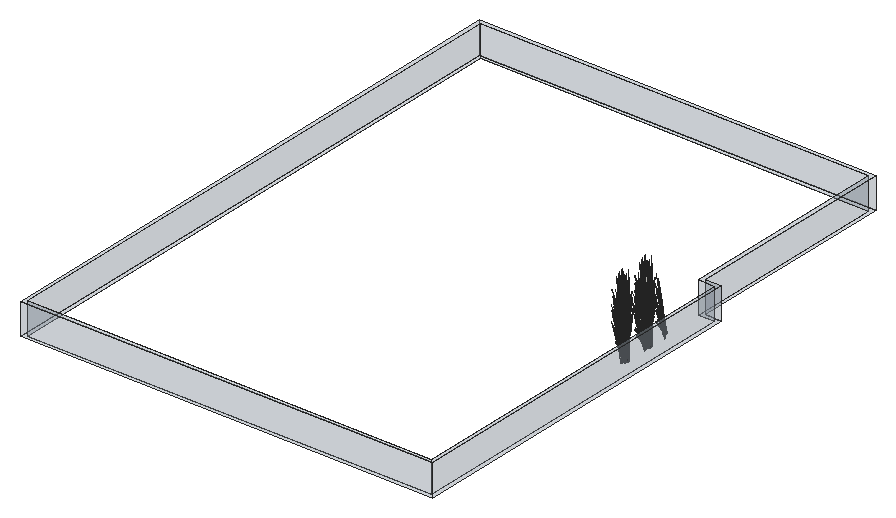
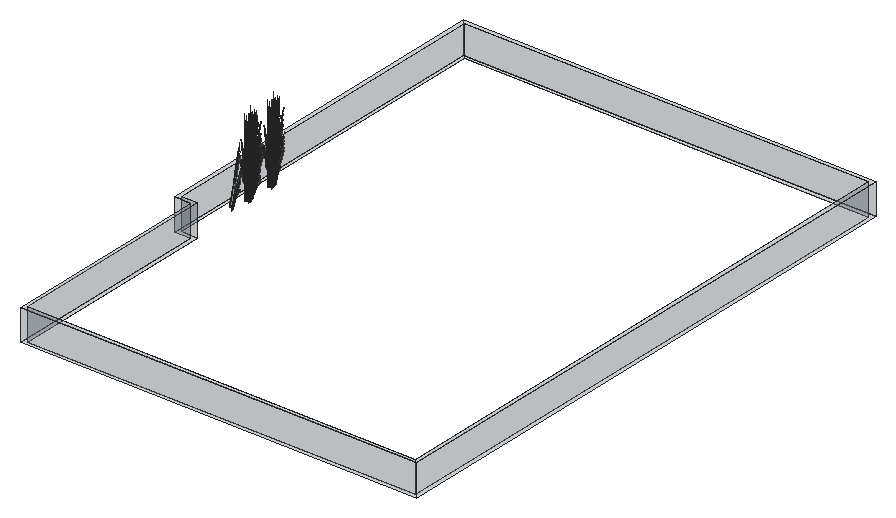
# SketchUp Ruby script. Lengths in inches.
U = 1.inch
M = Sketchup.active_model
def pt(a) = Geom::Point3d.new(a.map { |v| v * U })
def face(e, loops, mat)
  f = e.add_face(loops[0].map { |a| pt(a) })
  loops[1..].each { |l| e.add_face(l.map { |a| pt(a) }).erase! }
  f.material = f.back_material = mat if mat
  f
end
# faces: each face lists its corners as indices into pts; further lists are holes
def faces(e, pts, list, mat = nil) = list.each { |f| face(e, (f[0].is_a?(Array) ? f : [f]).map { |l| l.map { |i| pts[i] } }, mat) }
# xy, xz, yz: faces in a plane at the given z, y or x. An outline is a flat list of corners, or four numbers for a rectangle; further outlines are holes
def ring(l) = l.size == 4 ? [[l[0], l[1]], [l[2], l[1]], [l[2], l[3]], [l[0], l[3]]] : l.each_slice(2).to_a
def flat(e, list, mat, &to3) = list.each { |f| face(e, (f[0].is_a?(Array) ? f : [f]).map { |l| ring(l).map { |u, v| to3.(u, v) } }, mat) }
def xy(e, z, list, mat = nil) = flat(e, list, mat) { |x, y| [x, y, z] }
def xz(e, y, list, mat = nil) = flat(e, list, mat) { |x, z| [x, y, z] }
def yz(e, x, list, mat = nil) = flat(e, list, mat) { |y, z| [x, y, z] }
def lines(e, pts, list) = list.each { |a, b| e.add_line(pt(pts[a]), pt(pts[b])) }
# prism: a flat outline (further loops are holes) pulled along v
def prism(e, loops, v, mat = nil)
  f = face(e, loops, mat); d = Geom::Vector3d.new(v.map { |x| x * U })
  f.pushpull(f.normal.samedirection?(d) ? d.length : -d.length)
end
def box(e, o, s, mat = nil) = prism(e, [[o, [o[0] + s[0], o[1], o[2]], [o[0] + s[0], o[1] + s[1], o[2]], [o[0], o[1] + s[1], o[2]]]], [0, 0, s[2]], mat)
def at(x, y, z, deg = 0) = Geom::Transformation.translation(pt([x, y, z])) * Geom::Transformation.rotation(ORIGIN, Z_AXIS, deg.degrees)
def axes(o, x, y, z) = Geom::Transformation.new([*x, 0, *y, 0, *z, 0, *pt(o).to_a, 1])
def part(name) = M.definitions.add(name)
# library, detail: a bought-in or finely detailed component or shape, given as its bounding box
def library(name, o, s) = part(name).tap { |d| box(d.entities, o, s) }
def detail(e, o, s) = box(e.add_group.entities, o, s)
def put(e, d, t, mat = nil) = e.add_instance(d, t).tap { |i| i.material = mat if mat }
def group(e, t, mat = nil) = e.add_group.tap { |g| g.transformation = t; g.material = mat if mat }.entities
root = M.entities
M.materials.add("Glass_Basic_2").color = [161, 173, 186]
M.materials["Glass_Basic_2"].alpha = 0.25
M.materials.add("LightPink_Translucent").color = [144, 107, 117]
M.materials["LightPink_Translucent"].alpha = 0.75
c1 = part("blade")
p = [[2.15,0.21,22],[0,0.17,0],[0.09,0.45,0],[2.18,0.31,22],[2.29,0.31,22],[0.38,0.45,0],
  [2.48,0.24,33],[2.49,0.24,33],[2.48,0.22,33]]
faces(c1.entities,p,[[0,1,2,3],[4,5,2,3],[6,3,4,7],[8,0,3,6]])
c2 = part("seeds")
p = [[0.3,-0.1,1.38],[-0.01,-0.03,1.59],[-0.01,-0.03,0.03],[0.14,-0.07,-0.07],[0.29,-0.03,3],[0.15,0.01,3.11]]
faces(c2.entities,p,[[0,1,2,3],[1,0,4,5]],"LightPink_Translucent")
c3 = part("blade with seeds")
put(c3.entities,c1,at(0,0,0))
put(c3.entities,c2,axes([2.4,0.25,30.99],[1.5799,-0.05474,1.17369],[-0.12525,1.92788,0.29478],[-0.07173,-0.02425,1.56792]))
g1 = group(root,at(30.57,364.54,1398),"Glass_Basic_2")
prism(g1,[[[0,0,0],[0,434.16,0],[300,434.16,0],[300,273.36,0],[312,273.36,0],[312,0,0]],[[297,431.16,0],[3,431.16,0],[3,3,0],[309,3,0],[309,270.36,0],[297,270.36,0]]],[0,0,24])
put(root,c3,axes([329.46,560.04,1401.875],[0.14639,-0.01056,1.71376],[-0.09712,0.45778,0.13857],[-0.20862,-0.02831,0.73262]))
put(root,c3,axes([329.46,581.76,1401.875],[0.14639,-0.01056,1.71376],[-0.09712,0.45778,0.13857],[-0.20862,-0.02831,0.73262]))
put(root,c3,axes([329.52,560.85,1401.875],[0.12246,-0.09864,1.71376],[0.1031,0.45582,0.13857],[-0.19225,0.10302,0.73262]))
put(root,c3,axes([329.52,582.5625,1401.875],[0.12246,-0.09864,1.71376],[0.1031,0.45582,0.13857],[-0.19225,0.10302,0.73262]))
put(root,c3,axes([329.14,561.625,1400.59],[0.12266,0.03828,1.43002],[0.07906,0.39104,-0.30754],[-0.16661,0.0732,0.61141]))
put(root,c3,axes([329.14,583.34,1400.59],[0.12266,0.03828,1.43002],[0.07906,0.39104,-0.30754],[-0.16661,0.0732,0.61141]))
put(root,c3,axes([330.22,560.37,1401.34],[0.10032,-0.06746,1.77064],[0.0346,0.47103,0.13857],[-0.2173,0.0625,0.63284]))
put(root,c3,axes([330.22,582.09,1401.34],[0.10032,-0.06746,1.77064],[0.0346,0.47103,0.13857],[-0.2173,0.0625,0.63284]))
put(root,c3,axes([329.14,560.6875,1402.72],[-0.05763,0.06055,1.74944],[0.0049,0.44239,-0.27667],[-0.13211,0.05753,0.14031]))
put(root,c3,axes([329.14,582.4,1402.72],[-0.05763,0.06055,1.74944],[0.0049,0.44239,-0.27667],[-0.13211,0.05753,0.14031]))
put(root,c3,axes([329.89,559.62,1402.98],[-0.35281,-0.01123,-0.71045],[0.0237,-0.47284,0.08574],[-0.14947,-0.0499,1.00501]))
put(root,c3,axes([329.89,581.33,1402.98],[-0.35281,-0.01123,-0.71045],[0.0237,-0.47284,0.08574],[-0.14947,-0.0499,1.00501]))
put(root,c3,axes([329.61,559.73,1400.59],[0.06891,0.12984,1.43002],[-0.15879,0.35293,-0.30754],[-0.16304,-0.08436,0.61141]))
put(root,c3,axes([329.61,581.45,1400.59],[0.06891,0.12984,1.43002],[-0.15879,0.35293,-0.30754],[-0.16304,-0.08436,0.61141]))
put(root,c3,axes([329.33,560.43,1402.53],[-0.29332,-0.1301,-0.35414],[0.08555,-0.37955,0.4572],[-0.11809,0.0348,0.87481]))
put(root,c3,axes([329.33,582.15,1402.53],[-0.29332,-0.1301,-0.35414],[0.08555,-0.37955,0.4572],[-0.11809,0.0348,0.87481]))
put(root,c3,axes([329.73,581.02,1401.875],[0.1311,0.08035,1.71376],[-0.27131,0.33708,0.13857],[-0.16909,-0.15206,0.73262]))
put(root,c3,axes([328.5,561.13,1402.71],[0.04504,0.01251,1.77383],[0.13934,0.41205,-0.16761],[-0.0922,0.10815,0.31391]))
put(root,c3,axes([328.5,582.85,1402.71],[0.04504,0.01251,1.77383],[0.13934,0.41205,-0.16761],[-0.0922,0.10815,0.31391]))
put(root,c3,axes([329.53,560.63,1402.68],[-0.09562,0.42421,-0.51099],[-0.32782,-0.1454,-0.3958],[-0.13199,0.0389,0.97773]))
put(root,c3,axes([329.53,582.35,1402.68],[-0.09562,0.42421,-0.51099],[-0.32782,-0.1454,-0.3958],[-0.13199,0.0389,0.97773]))
put(root,c3,axes([329.78,559.71,1402.68],[-0.25628,0.30892,-0.51099],[-0.22444,-0.32634,-0.3958],[-0.13021,-0.047,0.97773]))
put(root,c3,axes([329.78,581.43,1402.68],[-0.25628,0.30892,-0.51099],[-0.22444,-0.32634,-0.3958],[-0.13021,-0.047,0.97773]))
put(root,c3,axes([329.36,560.6,1399.49],[0.00895,0.0735,1.76342],[-0.18044,0.38382,-0.26939],[-0.12817,-0.01935,0.30037]))
put(root,c3,axes([329.36,582.32,1399.49],[0.00895,0.0735,1.76342],[-0.18044,0.38382,-0.26939],[-0.12817,-0.01935,0.30037]))
put(root,c3,axes([329.42,558.85,1402.71],[0.02617,0.04654,1.77383],[-0.12614,0.41836,-0.16761],[-0.12775,0.00303,0.31391]))
put(root,c3,axes([329.42,580.5625,1402.71],[0.02617,0.04654,1.77383],[-0.12614,0.41836,-0.16761],[-0.12775,0.00303,0.31391]))
put(root,c3,axes([328.88,562.44,1400.77],[0.14709,-0.21136,1.1486],[0.05804,0.3346,0.84392],[-0.1063,0.05991,0.25299]))
put(root,c3,axes([328.88,584.16,1400.77],[0.14709,-0.21136,1.1486],[0.05804,0.3346,0.84392],[-0.1063,0.05991,0.25299]))
put(root,c3,axes([329.71,580.28,1402.72],[-0.07594,-0.00329,1.74944],[-0.24177,0.32918,-0.27667],[-0.129,-0.06726,0.14031]))
put(root,c3,axes([329.4,560.39,1402.73],[0.09971,-0.42522,0.48003],[0.32782,0.1454,0.3958],[-0.12892,0.02555,0.9933]))
put(root,c3,axes([329.4,582.1,1402.73],[0.09971,-0.42522,0.48003],[0.32782,0.1454,0.3958],[-0.12892,0.02555,0.9933]))
put(root,c3,axes([329.51,560.27,1403.03],[0.17758,0.42229,-0.1216],[-0.31518,0.20752,-0.67495],[-0.13282,0.05572,1.02557]))
put(root,c3,axes([329.51,581.98,1403.03],[0.17758,0.42229,-0.1216],[-0.31518,0.20752,-0.67495],[-0.13282,0.05572,1.02557]))
put(root,c3,axes([329.91,559.39,1403.03],[-0.0189,0.47427,-0.1216],[-0.35781,-0.01296,-0.67495],[-0.13781,-0.03295,1.02557]))
put(root,c3,axes([329.91,581.11,1403.03],[-0.0189,0.47427,-0.1216],[-0.35781,-0.01296,-0.67495],[-0.13781,-0.03295,1.02557]))
put(root,c3,axes([329.68,559.42,1402.53],[-0.20082,-0.29199,-0.35414],[0.2293,-0.2764,0.4572],[-0.1165,-0.04206,0.87481]))
put(root,c3,axes([329.68,581.14,1402.53],[-0.20082,-0.29199,-0.35414],[0.2293,-0.2764,0.4572],[-0.1165,-0.04206,0.87481]))
put(root,c3,axes([329.37,560.27,1402.73],[-0.12963,-0.31798,0.0643],[0.23638,-0.15564,0.50621],[-0.1042,0.03071,0.77189]))
put(root,c3,axes([329.37,581.99,1402.73],[-0.12963,-0.31798,0.0643],[0.23638,-0.15564,0.50621],[-0.1042,0.03071,0.77189]))
put(root,c3,axes([329.97,561.15,1401.875],[0.08815,-0.14329,1.71376],[0.22258,0.38678,0.13857],[-0.15267,0.17614,0.73262]))
put(root,c3,axes([329.97,582.87,1401.875],[0.08815,-0.14329,1.71376],[0.22258,0.38678,0.13857],[-0.15267,0.17614,0.73262]))
put(root,c3,axes([329.43,561.53,1402.53],[-0.30722,0.06665,-0.35414],[-0.08112,-0.381,0.4572],[-0.08804,0.10234,0.87481]))
put(root,c3,axes([329.43,583.25,1402.53],[-0.30722,0.06665,-0.35414],[-0.08112,-0.381,0.4572],[-0.08804,0.10234,0.87481]))
put(root,c3,axes([329.27,562.66,1399.49],[0.04734,0.04659,1.76342],[0.08027,0.4317,-0.26939],[-0.10492,0.09206,0.30037]))
put(root,c3,axes([329.27,584.38,1399.49],[0.04734,0.04659,1.76342],[0.08027,0.4317,-0.26939],[-0.10492,0.09206,0.30037]))
put(root,c3,axes([329.2,560.12,1400.77],[0.22533,-0.03337,1.1486],[-0.14293,0.29403,0.84392],[-0.11135,-0.04411,0.25299]))
put(root,c3,axes([329.2,581.84,1400.77],[0.22533,-0.03337,1.1486],[-0.14293,0.29403,0.84392],[-0.11135,-0.04411,0.25299]))
put(root,c3,axes([329.47,561.45,1402.73],[-0.08753,-0.42921,0.48003],[0.34336,-0.07449,0.3958],[-0.1012,0.10094,0.9933]))
put(root,c3,axes([329.47,583.16,1402.73],[-0.08753,-0.42921,0.48003],[0.34336,-0.07449,0.3958],[-0.1012,0.10094,0.9933]))
put(root,c3,axes([329.65,559.3125,1403.09],[0.29147,-0.34417,0.53763],[0.25138,0.3655,0.4433],[-0.13675,-0.06349,1.11249]))
put(root,c3,axes([329.65,581.03,1403.09],[0.29147,-0.34417,0.53763],[0.25138,0.3655,0.4433],[-0.13675,-0.06349,1.11249]))
put(root,c3,axes([329.41,561.36,1402.73],[-0.2423,-0.19613,0.0643],[0.14107,-0.2793,0.50621],[-0.07768,0.0903,0.77189]))
put(root,c3,axes([329.41,583.08,1402.73],[-0.2423,-0.19613,0.0643],[0.14107,-0.2793,0.50621],[-0.07768,0.0903,0.77189]))
put(root,c3,axes([329.9,561.51,1401.875],[0.06572,-0.16029,1.71376],[0.27569,0.33172,0.13857],[-0.12437,0.20675,0.73262]))
put(root,c3,axes([329.9,583.22,1401.875],[0.06572,-0.16029,1.71376],[0.27569,0.33172,0.13857],[-0.12437,0.20675,0.73262]))
put(root,c3,axes([329.64,560.39,1403.05],[0.29332,0.1301,0.35414],[-0.08555,0.37955,-0.4572],[-0.11809,0.0348,0.87481]))
put(root,c3,axes([329.64,582.11,1403.05],[0.29332,0.1301,0.35414],[-0.08555,0.37955,-0.4572],[-0.11809,0.0348,0.87481]))
put(root,c3,axes([329.6875,561.57,1402.68],[0.09067,0.42583,-0.51099],[-0.34336,0.07449,-0.3958],[-0.0984,0.11438,0.97773]))
put(root,c3,axes([329.6875,583.29,1402.68],[0.09067,0.42583,-0.51099],[-0.34336,0.07449,-0.3958],[-0.0984,0.11438,0.97773]))
put(root,c3,axes([329.78,559.31,1402.73],[0.01777,-0.35463,0.0643],[0.26836,0.00972,0.50621],[-0.1028,-0.03711,0.77189]))
put(root,c3,axes([329.78,581.03,1402.73],[0.01777,-0.35463,0.0643],[0.26836,0.00972,0.50621],[-0.1028,-0.03711,0.77189]))
put(root,c3,axes([329.15,562.34,1402.72],[-0.00877,0.09229,1.74944],[0.24897,0.32105,-0.27667],[-0.06518,0.15182,0.14031]))
put(root,c3,axes([329.15,584.06,1402.72],[-0.00877,0.09229,1.74944],[0.24897,0.32105,-0.27667],[-0.06518,0.15182,0.14031]))
put(root,c3,axes([330.54,561.27,1400.06],[-0.36714,-0.07646,-0.62353],[0.07747,-0.47163,-0.16365],[-0.10956,-0.05715,1.37633]))
put(root,c3,axes([330.54,582.99,1400.06],[-0.36714,-0.07646,-0.62353],[0.07747,-0.47163,-0.16365],[-0.10956,-0.05715,1.37633]))
put(root,c3,axes([330.61,580.41,1403.43],[-0.23555,0.44708,-0.13619],[-0.34112,-0.25757,-0.75594],[-0.11858,-0.12631,1.14864]))
put(root,c3,axes([329.97,559.57,1403.05],[0.20082,0.29199,0.35414],[-0.2293,0.2764,-0.4572],[-0.1165,-0.04206,0.87481]))
put(root,c3,axes([329.97,581.29,1403.05],[0.20082,0.29199,0.35414],[-0.2293,0.2764,-0.4572],[-0.1165,-0.04206,0.87481]))
put(root,c3,axes([330.51,580.78,1402.98],[-0.30095,-0.22541,-0.71045],[0.21388,-0.395,0.08574],[-0.10904,-0.13459,1.00501]))
put(root,c3,axes([330.37,580.79,1402.68],[-0.34827,0.11086,-0.51099],[-0.06092,-0.41983,-0.3958],[-0.09354,-0.12031,0.97773]))
put(root,c3,axes([330.0625,562.16,1400.02],[-0.33032,-0.23318,-0.49651],[0.19744,-0.41812,0],[-0.07523,-0.05311,1.57504]))
put(root,c3,axes([330.0625,583.88,1400.02],[-0.33032,-0.23318,-0.49651],[0.19744,-0.41812,0],[-0.07523,-0.05311,1.57504]))
put(root,c3,axes([329.92,580.4,1399.49],[-0.03419,0.06144,1.76342],[-0.3455,0.13246,-0.26939],[-0.08346,-0.12049,0.30037]))
put(root,c3,axes([329.53,561.27,1403.03],[0.32648,0.25715,-0.1216],[-0.18809,0.3724,-0.67495],[-0.09224,0.12945,1.02557]))
put(root,c3,axes([329.53,582.99,1403.03],[0.32648,0.25715,-0.1216],[-0.18809,0.3724,-0.67495],[-0.09224,0.12945,1.02557]))
put(root,c3,axes([330.26,562.44,1400.375],[-0.22066,0.46731,0],[-0.36918,-0.26061,-0.51607],[-0.08408,-0.05936,1.63711]))
put(root,c3,axes([330.26,584.16,1400.375],[-0.22066,0.46731,0],[-0.36918,-0.26061,-0.51607],[-0.08408,-0.05936,1.63711]))
put(root,c3,axes([328.99,562.39,1403.65],[0.31145,0.12449,-0.06488],[-0.0958,0.38314,-0.29416],[-0.05094,0.05817,0.97024]))
put(root,c3,axes([328.99,584.1,1403.65],[0.31145,0.12449,-0.06488],[-0.0958,0.38314,-0.29416],[-0.05094,0.05817,0.97024]))
put(root,c3,axes([329.6875,561.3,1403.05],[0.30722,-0.06665,0.35414],[0.08112,0.381,-0.4572],[-0.08804,0.10234,0.87481]))
put(root,c3,axes([329.6875,583.02,1403.05],[0.30722,-0.06665,0.35414],[0.08112,0.381,-0.4572],[-0.08804,0.10234,0.87481]))
put(root,c3,axes([329.86,563.12,1400.59],[0.11138,-0.07357,1.43002],[0.27499,0.22183,-0.30754],[-0.08185,0.19194,0.61141]))
put(root,c3,axes([329.86,584.84,1400.59],[0.11138,-0.07357,1.43002],[0.27499,0.22183,-0.30754],[-0.08185,0.19194,0.61141]))
put(root,c3,axes([329.7,558.92,1400.13],[-0.10181,0.3808,-0.03893],[-0.31336,-0.11714,-0.17649],[-0.04758,-0.06228,0.58215]))
put(root,c3,axes([329.7,580.64,1400.13],[-0.10181,0.3808,-0.03893],[-0.31336,-0.11714,-0.17649],[-0.04758,-0.06228,0.58215]))
put(root,c3,axes([330.52,579.35,1402.71],[-0.00658,0.0559,1.77383],[-0.32474,0.20287,-0.16761],[-0.09556,-0.1037,0.31391]))
put(root,c3,axes([330.52,598.27,1402.71],[-0.00658,0.0559,1.77383],[-0.32474,0.20287,-0.16761],[-0.09556,-0.1037,0.31391]))
put(root,c3,axes([330.17,580.16,1400.59],[-0.02137,0.15256,1.43002],[-0.31245,0.12771,-0.30754],[-0.07303,-0.19719,0.61141]))
put(root,c3,axes([330.17,599.08,1400.59],[-0.02137,0.15256,1.43002],[-0.31245,0.12771,-0.30754],[-0.07303,-0.19719,0.61141]))
put(root,c3,axes([330.27,580.56,1401.875],[0.08068,0.14973,1.71376],[-0.3728,0.12606,0.13857],[-0.08426,-0.23506,0.73262]))
put(root,c3,axes([330.27,599.47,1401.875],[0.08068,0.14973,1.71376],[-0.3728,0.12606,0.13857],[-0.08426,-0.23506,0.73262]))
put(root,c3,axes([330.96,561.34,1400.67],[-0.35635,0.30962,-0.29095],[-0.23697,-0.43749,-0.50002],[-0.08792,-0.04443,1.59708]))
put(root,c3,axes([330.96,583.06,1400.67],[-0.35635,0.30962,-0.29095],[-0.23697,-0.43749,-0.50002],[-0.08792,-0.04443,1.59708]))
put(root,c3,axes([329.98,562.32,1402.73],[-0.25132,-0.3182,0.48003],[0.2669,-0.27442,0.3958],[-0.04636,0.14929,0.9933]))
put(root,c3,axes([329.98,584.03,1402.73],[-0.25132,-0.3182,0.48003],[0.2669,-0.27442,0.3958],[-0.04636,0.14929,0.9933]))
put(root,c3,axes([330.4,580.48,1402.53],[-0.05451,-0.37564,-0.35414],[0.31161,-0.09919,0.4572],[-0.0837,-0.10765,0.87481]))
put(root,c3,axes([329.53,560.66,1400.375],[-0.44133,0,0],[0,-0.52122,-0.51607],[0,-0.11871,1.63711]))
put(root,c3,axes([329.53,582.38,1400.375],[-0.44133,0,0],[0,-0.52122,-0.51607],[0,-0.11871,1.63711]))
put(root,c3,axes([330.15,561.99,1400.03],[-0.08291,-0.40636,-0.30978],[0.32928,-0.11539,0.30978],[-0.06638,-0.04686,1.38974]))
put(root,c3,axes([330.15,583.7,1400.03],[-0.08291,-0.40636,-0.30978],[0.32928,-0.11539,0.30978],[-0.06638,-0.04686,1.38974]))
put(root,c3,axes([329.88,562.29,1402.73],[-0.29004,-0.02173,0.0643],[0.00795,-0.32812,0.50621],[-0.03035,0.12569,0.77189]))
put(root,c3,axes([329.88,584,1402.73],[-0.29004,-0.02173,0.0643],[0.00795,-0.32812,0.50621],[-0.03035,0.12569,0.77189]))
put(root,c3,axes([329.98,562.41,1402.53],[-0.23881,0.24554,-0.35414],[-0.22606,-0.28036,0.4572],[-0.0344,0.14245,0.87481]))
put(root,c3,axes([329.98,584.13,1402.53],[-0.23881,0.24554,-0.35414],[-0.22606,-0.28036,0.4572],[-0.0344,0.14245,0.87481]))
put(root,c3,axes([331.2,561.68,1400.06],[-0.23773,0.35053,-0.62353],[-0.29532,-0.31785,-0.16365],[-0.09526,0.08744,1.37633]))
put(root,c3,axes([331.2,583.39,1400.06],[-0.23773,0.35053,-0.62353],[-0.29532,-0.31785,-0.16365],[-0.09526,0.08744,1.37633]))
put(root,c3,axes([330.59,559.07,1403.05],[0.05451,0.37564,0.35414],[-0.31161,0.09919,-0.4572],[-0.0837,-0.10765,0.87481]))
put(root,c3,axes([330.59,580.78,1403.05],[0.05451,0.37564,0.35414],[-0.31161,0.09919,-0.4572],[-0.0837,-0.10765,0.87481]))
put(root,c3,axes([329.125,563.28,1402.71],[0.04004,-0.02816,1.77383],[0.33095,0.18728,-0.16761],[-0.00778,0.15594,0.31391]))
put(root,c3,axes([329.125,585,1402.71],[0.04004,-0.02816,1.77383],[0.33095,0.18728,-0.16761],[-0.00778,0.15594,0.31391]))
put(root,c3,axes([329.875,560.52,1400.33],[-0.32829,0.39208,0.30756],[-0.32849,-0.38796,-0.36492],[-0.01146,-0.11134,1.64885]))
put(root,c3,axes([329.875,582.24,1400.33],[-0.32829,0.39208,0.30756],[-0.32849,-0.38796,-0.36492],[-0.01146,-0.11134,1.64885]))
put(root,c3,axes([331.23,561.61,1401.33],[0.305,0.18805,1.51261],[-0.29879,0.40513,0.59816],[-0.13384,-0.24012,1.26806]))
put(root,c3,axes([331.23,583.33,1401.33],[0.305,0.18805,1.51261],[-0.29879,0.40513,0.59816],[-0.13384,-0.24012,1.26806]))
put(root,c3,axes([330.0625,579.92,1400.77],[0.18411,0.16231,1.1486],[-0.26813,0.09757,0.84392],[-0.05737,-0.12474,0.25299]))
put(root,c3,axes([330.0625,598.83,1400.77],[0.18411,0.16231,1.1486],[-0.26813,0.09757,0.84392],[-0.05737,-0.12474,0.25299]))
put(root,c3,axes([331.36,561.48,1400.46],[-0.34464,-0.37536,-0.25192],[0.29,-0.42149,0.5513],[-0.0928,0.04391,1.68216]))
put(root,c3,axes([331.36,583.2,1400.46],[-0.34464,-0.37536,-0.25192],[0.29,-0.42149,0.5513],[-0.0928,0.04391,1.68216]))
put(root,c3,axes([330.73,561.12,1400.21],[-0.21202,-0.39143,-0.44739],[0.32115,-0.27564,0.21531],[-0.06861,-0.04843,1.43643]))
put(root,c3,axes([330.73,582.84,1400.21],[-0.21202,-0.39143,-0.44739],[0.32115,-0.27564,0.21531],[-0.06861,-0.04843,1.43643]))
put(root,c3,axes([330.13,562.15,1403.34],[-0.00918,0.43138,-0.7886],[-0.38672,-0.02897,0.09517],[-0.04081,0.18275,1.11556]))
put(root,c3,axes([330.13,583.87,1403.34],[-0.00918,0.43138,-0.7886],[-0.38672,-0.02897,0.09517],[-0.04081,0.18275,1.11556]))
put(root,c3,axes([330.13,563.36,1400.77],[-0.00913,-0.2773,1.1486],[0.22824,0.19778,0.84392],[-0.04489,0.13217,0.25299]))
put(root,c3,axes([330.13,585.08,1400.77],[-0.00913,-0.2773,1.1486],[0.22824,0.19778,0.84392],[-0.04489,0.13217,0.25299]))
put(root,c3,axes([330.45,580.34,1403.09],[0.39316,-0.11987,0.53763],[0.06823,0.47021,0.4433],[-0.09247,-0.13858,1.11249]))
put(root,c3,axes([330.45,599.26,1403.09],[0.39316,-0.11987,0.53763],[0.06823,0.47021,0.4433],[-0.09247,-0.13858,1.11249]))
put(root,c3,axes([331.1875,561.4,1400.21],[-0.38326,0.02879,-0.44739],[-0.03466,-0.47788,0.21531],[-0.06861,0.04843,1.43643]))
put(root,c3,axes([331.1875,583.12,1400.21],[-0.38326,0.02879,-0.44739],[-0.03466,-0.47788,0.21531],[-0.06861,0.04843,1.43643]))
put(root,c3,axes([330.54,580.44,1402.73],[0.16041,-0.29625,0.0643],[0.22843,0.17248,0.50621],[-0.07385,-0.09498,0.77189]))
put(root,c3,axes([330.45,562.2,1400.48],[0.33032,0.23318,0.49651],[-0.19744,0.41812,0],[-0.07523,-0.05311,1.57504]))
put(root,c3,axes([330.45,583.92,1400.48],[0.33032,0.23318,0.49651],[-0.19744,0.41812,0],[-0.07523,-0.05311,1.57504]))
put(root,c3,axes([330.01,562.76,1401.36],[0.00775,-0.24075,1.54345],[0.34877,0.12716,0.21329],[-0.03022,0.25658,0.72882]))
put(root,c3,axes([330.01,584.48,1401.36],[0.00775,-0.24075,1.54345],[0.34877,0.12716,0.21329],[-0.03022,0.25658,0.72882]))
put(root,c3,axes([330.77,561.34,1400.4375],[0.09355,-0.55261,-0.23429],[0.44354,0.09633,0.51271],[-0.0775,-0.07631,1.5644]))
put(root,c3,axes([330.77,583.06,1400.4375],[0.09355,-0.55261,-0.23429],[0.44354,0.09633,0.51271],[-0.0775,-0.07631,1.5644]))
put(root,c3,axes([330.93,561.47,1400.62],[-0.06809,0.4162,0.1448],[-0.33266,-0.07225,-0.41347],[-0.06054,-0.04274,1.26744]))
put(root,c3,axes([330.93,583.19,1400.62],[-0.06809,0.4162,0.1448],[-0.33266,-0.07225,-0.41347],[-0.06054,-0.04274,1.26744]))
put(root,c3,axes([330.89,579.5625,1402.72],[-0.05398,-0.06539,1.74944],[-0.36026,0.04145,-0.27667],[-0.0575,-0.15639,0.14031]))
put(root,c3,axes([330.89,598.48,1402.72],[-0.05398,-0.06539,1.74944],[-0.36026,0.04145,-0.27667],[-0.0575,-0.15639,0.14031]))
put(root,c3,axes([331.59,562.63,1400.02],[-0.33032,0.23318,-0.49651],[-0.19744,-0.41812,0],[-0.07523,0.05311,1.57504]))
put(root,c3,axes([331.59,584.35,1400.02],[-0.33032,0.23318,-0.49651],[-0.19744,-0.41812,0],[-0.07523,0.05311,1.57504]))
put(root,c3,axes([329.63,560.31,1400.02],[0,-0.46636,-0.49651],[0.39487,0,0],[0,-0.10622,1.57504]))
put(root,c3,axes([329.63,582.03,1400.02],[0,-0.46636,-0.49651],[0.39487,0,0],[0,-0.10622,1.57504]))
put(root,c3,axes([329.8,560.74,1400.48],[0,0.46636,0.49651],[-0.39487,0,0],[0,-0.10622,1.57504]))
put(root,c3,axes([329.8,582.46,1400.48],[0,0.46636,0.49651],[-0.39487,0,0],[0,-0.10622,1.57504]))
put(root,c3,axes([331.61,562.51,1400.19],[-0.21791,-0.46895,-0.05142],[0.36918,-0.26061,0.51607],[-0.09097,0.04465,1.6363]))
put(root,c3,axes([331.61,584.22,1400.19],[-0.21791,-0.46895,-0.05142],[0.36918,-0.26061,0.51607],[-0.09097,0.04465,1.6363]))
put(root,c3,axes([330.21,562.29,1403],[0.25266,0.31335,-0.5672],[-0.2669,0.27442,-0.43934],[-0.03844,0.15921,1.08528]))
put(root,c3,axes([330.21,584.01,1403],[0.25266,0.31335,-0.5672],[-0.2669,0.27442,-0.43934],[-0.03844,0.15921,1.08528]))
put(root,c3,axes([331.51,562.45,1400.03],[-0.32928,-0.11539,-0.30978],[0.08291,-0.40636,0.30978],[-0.06638,0.04686,1.38974]))
put(root,c3,axes([331.51,584.17,1400.03],[-0.32928,-0.11539,-0.30978],[0.08291,-0.40636,0.30978],[-0.06638,0.04686,1.38974]))
put(root,c3,axes([330.1,562.0625,1403.05],[0.23881,-0.24554,0.35414],[0.22606,0.28036,-0.4572],[-0.0344,0.14245,0.87481]))
put(root,c3,axes([330.1,583.78,1403.05],[0.23881,-0.24554,0.35414],[0.22606,0.28036,-0.4572],[-0.0344,0.14245,0.87481]))
put(root,c3,axes([330.67,560.85,1400.67],[-0.39748,-0.22252,-0.29095],[0.19139,-0.46966,-0.50002],[-0.01249,-0.11531,1.59708]))
put(root,c3,axes([330.67,582.57,1400.67],[-0.39748,-0.22252,-0.29095],[0.19139,-0.46966,-0.50002],[-0.01249,-0.11531,1.59708]))
put(root,c3,axes([331.7,560.71,1400.84],[-0.00964,-0.43909,1.41272],[0.43635,0.11382,0.59816],[-0.1032,0.24027,1.3335]))
put(root,c3,axes([331.7,582.43,1400.84],[-0.00964,-0.43909,1.41272],[0.43635,0.11382,0.59816],[-0.1032,0.24027,1.3335]))
put(root,c3,axes([329.95,562.13,1403.4],[0.3879,0.02311,-0.13498],[-0.0106,0.43749,-0.74919],[-0.02694,0.1685,1.13838]))
put(root,c3,axes([329.95,583.85,1403.4],[0.3879,0.02311,-0.13498],[-0.0106,0.43749,-0.74919],[-0.02694,0.1685,1.13838]))
put(root,c3,axes([329.9375,562.77,1400.82],[0.32063,-0.08258,0.06507],[0.07371,0.33271,-0.86304],[-0.02033,0.16842,0.7736]))
put(root,c3,axes([329.9375,584.48,1400.82],[0.32063,-0.08258,0.06507],[0.07371,0.33271,-0.86304],[-0.02033,0.16842,0.7736]))
put(root,c3,axes([331.46,561.27,1400.67],[0.04113,0.53214,-0.29095],[-0.42835,0.03218,-0.50002],[-0.07543,0.07088,1.59708]))
put(root,c3,axes([331.46,582.99,1400.67],[0.04113,0.53214,-0.29095],[-0.42835,0.03218,-0.50002],[-0.07543,0.07088,1.59708]))
put(root,c3,axes([330.49,582.09,1400.1],[-0.14494,-0.47823,-0.69835],[0.41752,-0.17223,-0.18329],[-0.01602,-0.16194,1.54149]))
put(root,c3,axes([331.4375,580.57,1403.03],[-0.34538,0.21713,-0.1216],[-0.16972,-0.38536,-0.67495],[-0.04557,-0.16239,1.02557]))
put(root,c3,axes([331.4375,599.49,1403.03],[-0.34538,0.21713,-0.1216],[-0.16972,-0.38536,-0.67495],[-0.04557,-0.16239,1.02557]))
put(root,c3,axes([331.14,580.59,1402.68],[-0.34695,-0.11691,-0.51099],[0.11892,-0.40083,-0.3958],[-0.03181,-0.16138,0.97773]))
put(root,c3,axes([331.14,599.51,1402.68],[-0.34695,-0.11691,-0.51099],[0.11892,-0.40083,-0.3958],[-0.03181,-0.16138,0.97773]))
put(root,c3,axes([330.5,561.85,1401.875],[-0.00864,-0.17899,1.71376],[0.37441,0.11874,0.13857],[-0.02316,0.25508,0.73262]))
put(root,c3,axes([330.5,583.5625,1401.875],[-0.00864,-0.17899,1.71376],[0.37441,0.11874,0.13857],[-0.02316,0.25508,0.73262]))
put(root,c3,axes([329.8,560.32,1400.03],[0.24637,-0.29097,-0.30978],[0.24637,0.29097,0.30978],[0,-0.09372,1.38974]))
put(root,c3,axes([329.8,582.04,1400.03],[0.24637,-0.29097,-0.30978],[0.24637,0.29097,0.30978],[0,-0.09372,1.38974]))
put(root,c3,axes([330.92,580.15,1400.13],[-0.2439,0.26754,-0.03893],[-0.22348,-0.29302,-0.17649],[-0.01573,-0.08303,0.58215]))
put(root,c3,axes([330.82,561.08,1400.36],[0.44609,0.09826,0.45755],[-0.09078,0.55493,0.17955],[-0.06519,-0.05359,1.58856]))
put(root,c3,axes([330.82,582.79,1400.36],[0.44609,0.09826,0.45755],[-0.09078,0.55493,0.17955],[-0.06519,-0.05359,1.58856]))
put(root,c3,axes([330.7,560.98,1400.72],[-0.17124,0.42022,0.44739],[-0.35581,-0.20224,-0.21531],[0,-0.09687,1.43643]))
put(root,c3,axes([330.7,582.69,1400.72],[-0.17124,0.42022,0.44739],[-0.35581,-0.20224,-0.21531],[0,-0.09687,1.43643]))
put(root,c3,axes([331.27,580.67,1402.98],[-0.16845,-0.3792,-0.71045],[0.34676,-0.21133,0.08574],[-0.03939,-0.18322,1.00501]))
put(root,c3,axes([331.27,599.59,1402.98],[-0.16845,-0.3792,-0.71045],[0.34676,-0.21133,0.08574],[-0.03939,-0.18322,1.00501]))
put(root,c3,axes([330.58,561.96,1400.47],[0.37926,-0.12378,0.17642],[0.09365,0.46065,0.35086],[-0.03382,-0.06712,1.60407]))
put(root,c3,axes([330.58,583.68,1400.47],[0.37926,-0.12378,0.17642],[0.09365,0.46065,0.35086],[-0.03382,-0.06712,1.60407]))
put(root,c3,axes([331.07,562.04,1400.2],[-0.35581,-0.20937,0],[0.17124,-0.43505,0],[0,0,1.62707]))
put(root,c3,axes([331.07,583.75,1400.2],[-0.35581,-0.20937,0],[0.17124,-0.43505,0],[0,0,1.62707]))
put(root,c3,axes([331.33,580.72,1403.05],[-0.1064,0.35863,0.35414],[-0.31043,-0.1046,-0.4572],[-0.02846,-0.14439,0.87481]))
put(root,c3,axes([331.89,562.56,1400.375],[0.22066,0.46731,0],[-0.36918,0.26061,-0.51607],[-0.08408,0.05936,1.63711]))
put(root,c3,axes([331.89,584.28,1400.375],[0.22066,0.46731,0],[-0.36918,0.26061,-0.51607],[-0.08408,0.05936,1.63711]))
put(root,c3,axes([330.77,562.76,1403.0625],[-0.34777,-0.12192,0.53283],[0.11892,-0.40083,0.43934],[0.0209,0.15763,1.10256]))
put(root,c3,axes([330.77,584.48,1403.0625],[-0.34777,-0.12192,0.53283],[0.11892,-0.40083,0.43934],[0.0209,0.15763,1.10256]))
put(root,c3,axes([330.67,562.79,1402.73],[-0.26007,0.1585,0.0643],[-0.12729,-0.28902,0.50621],[0.02512,0.1274,0.77189]))
put(root,c3,axes([330.67,584.51,1402.73],[-0.26007,0.1585,0.0643],[-0.12729,-0.28902,0.50621],[0.02512,0.1274,0.77189]))
put(root,c3,axes([331.71,561.99,1400.47],[0.10196,-0.46348,0.17642],[0.3731,0.13116,0.35086],[-0.06445,0.00226,1.60407]))
put(root,c3,axes([331.71,583.71,1400.47],[0.10196,-0.46348,0.17642],[0.3731,0.13116,0.35086],[-0.06445,0.00226,1.60407]))
put(root,c3,axes([331.53,561.37,1400.62],[0.26075,0.2802,0.1448],[-0.2175,0.31612,-0.41347],[-0.06054,0.04274,1.26744]))
put(root,c3,axes([331.53,583.09,1400.62],[0.26075,0.2802,0.1448],[-0.2175,0.31612,-0.41347],[-0.06054,0.04274,1.26744]))
put(root,c3,axes([331.44,561.03,1400.3],[-0.32829,-0.4014,-0.06131],[0.32849,-0.40164,0],[-0.01146,-0.01402,1.75571]))
put(root,c3,axes([331.44,582.74,1400.3],[-0.32829,-0.4014,-0.06131],[0.32849,-0.40164,0],[-0.01146,-0.01402,1.75571]))
put(root,c3,axes([331.53,561.17,1400.72],[0.38326,-0.02879,0.44739],[0.03466,0.47788,-0.21531],[-0.06861,0.04843,1.43643]))
put(root,c3,axes([331.53,582.88,1400.72],[0.38326,-0.02879,0.44739],[0.03466,0.47788,-0.21531],[-0.06861,0.04843,1.43643]))
put(root,c3,axes([331.62,562.27,1400.33],[0.44186,0.15158,0.30756],[-0.11054,0.54181,-0.36492],[-0.07313,0.06781,1.64885]))
put(root,c3,axes([331.62,583.98,1400.33],[0.44186,0.15158,0.30756],[-0.11054,0.54181,-0.36492],[-0.07313,0.06781,1.64885]))
put(root,c3,axes([330.98,579.83,1399.49],[-0.0592,0.0168,1.76342],[-0.32738,-0.18913,-0.26939],[0.00549,-0.15776,0.30037]))
put(root,c3,axes([330.98,598.74,1399.49],[-0.0592,0.0168,1.76342],[-0.32738,-0.18913,-0.26939],[0.00549,-0.15776,0.30037]))
put(root,c3,axes([331.8125,562.24,1400.48],[0.33032,-0.23318,0.49651],[0.19744,0.41812,0],[-0.07523,0.05311,1.57504]))
put(root,c3,axes([331.8125,583.95,1400.48],[0.33032,-0.23318,0.49651],[0.19744,0.41812,0],[-0.07523,0.05311,1.57504]))
put(root,c3,axes([331.3,580.35,1402.53],[0.1064,-0.35863,-0.35414],[0.31043,0.1046,0.4572],[-0.02846,-0.14439,0.87481]))
put(root,c3,axes([331.3,599.26,1402.53],[0.1064,-0.35863,-0.35414],[0.31043,0.1046,0.4572],[-0.02846,-0.14439,0.87481]))
put(root,c3,axes([330.78,560.57,1400.36],[0.15345,0.52148,0.45755],[-0.43845,0.18134,0.17955],[0.00536,-0.09582,1.58856]))
put(root,c3,axes([330.78,582.28,1400.36],[0.15345,0.52148,0.45755],[-0.43845,0.18134,0.17955],[0.00536,-0.09582,1.58856]))
